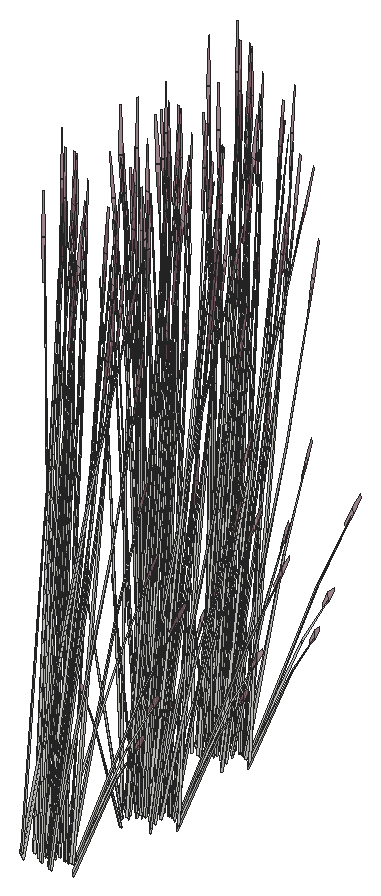
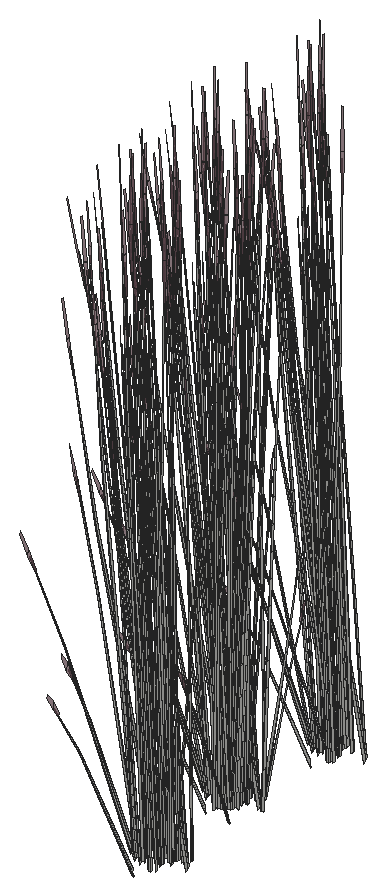
# SketchUp Ruby script. Lengths in inches.
U = 1.inch
M = Sketchup.active_model
def pt(a) = Geom::Point3d.new(a.map { |v| v * U })
def face(e, loops, mat)
  f = e.add_face(loops[0].map { |a| pt(a) })
  loops[1..].each { |l| e.add_face(l.map { |a| pt(a) }).erase! }
  f.material = f.back_material = mat if mat
  f
end
# faces: each face lists its corners as indices into pts; further lists are holes
def faces(e, pts, list, mat = nil) = list.each { |f| face(e, (f[0].is_a?(Array) ? f : [f]).map { |l| l.map { |i| pts[i] } }, mat) }
# xy, xz, yz: faces in a plane at the given z, y or x. An outline is a flat list of corners, or four numbers for a rectangle; further outlines are holes
def ring(l) = l.size == 4 ? [[l[0], l[1]], [l[2], l[1]], [l[2], l[3]], [l[0], l[3]]] : l.each_slice(2).to_a
def flat(e, list, mat, &to3) = list.each { |f| face(e, (f[0].is_a?(Array) ? f : [f]).map { |l| ring(l).map { |u, v| to3.(u, v) } }, mat) }
def xy(e, z, list, mat = nil) = flat(e, list, mat) { |x, y| [x, y, z] }
def xz(e, y, list, mat = nil) = flat(e, list, mat) { |x, z| [x, y, z] }
def yz(e, x, list, mat = nil) = flat(e, list, mat) { |y, z| [x, y, z] }
def lines(e, pts, list) = list.each { |a, b| e.add_line(pt(pts[a]), pt(pts[b])) }
# prism: a flat outline (further loops are holes) pulled along v
def prism(e, loops, v, mat = nil)
  f = face(e, loops, mat); d = Geom::Vector3d.new(v.map { |x| x * U })
  f.pushpull(f.normal.samedirection?(d) ? d.length : -d.length)
end
def box(e, o, s, mat = nil) = prism(e, [[o, [o[0] + s[0], o[1], o[2]], [o[0] + s[0], o[1] + s[1], o[2]], [o[0], o[1] + s[1], o[2]]]], [0, 0, s[2]], mat)
def at(x, y, z, deg = 0) = Geom::Transformation.translation(pt([x, y, z])) * Geom::Transformation.rotation(ORIGIN, Z_AXIS, deg.degrees)
def axes(o, x, y, z) = Geom::Transformation.new([*x, 0, *y, 0, *z, 0, *pt(o).to_a, 1])
def part(name) = M.definitions.add(name)
# library, detail: a bought-in or finely detailed component or shape, given as its bounding box
def library(name, o, s) = part(name).tap { |d| box(d.entities, o, s) }
def detail(e, o, s) = box(e.add_group.entities, o, s)
def put(e, d, t, mat = nil) = e.add_instance(d, t).tap { |i| i.material = mat if mat }
def group(e, t, mat = nil) = e.add_group.tap { |g| g.transformation = t; g.material = mat if mat }.entities
root = M.entities
M.materials.add("LightPink_Translucent").color = [144, 107, 117]
M.materials["LightPink_Translucent"].alpha = 0.75
c1 = part("blade")
p = [[2.15,0.21,22],[0,0.17,0],[0.09,0.45,0],[2.18,0.31,22],[2.29,0.31,22],[0.38,0.45,0],
  [2.48,0.24,33],[2.49,0.24,33],[2.48,0.22,33]]
faces(c1.entities,p,[[0,1,2,3],[4,5,2,3],[6,3,4,7],[8,0,3,6]])
c2 = part("seeds")
p = [[0.3,-0.1,1.38],[-0.01,-0.03,1.59],[-0.01,-0.03,0.03],[0.14,-0.07,-0.07],[0.29,-0.03,3],[0.15,0.01,3.11]]
faces(c2.entities,p,[[0,1,2,3],[1,0,4,5]],"LightPink_Translucent")
c3 = part("blade with seeds")
put(c3.entities,c1,at(0,0,0))
put(c3.entities,c2,axes([2.4,0.25,30.99],[1.5799,-0.05474,1.17369],[-0.12525,1.92788,0.29478],[-0.07173,-0.02425,1.56792]))
put(root,c3,axes([334.97,422.4,50.19],[-0.47255,-0.19538,0.43871],[0.28245,-0.35034,0],[0.10763,0.0445,1.3917]))
put(root,c3,axes([333.91,423.16,50.09],[-0.41865,0.35461,0.40429],[-0.49737,-0.31303,0.15865],[0.10093,-0.03539,1.40366]))
put(root,c3,axes([333.18,422.58,50.1875],[-0.14586,0.38834,0.15589],[-0.53375,-0.1099,0.31002],[0.0922,-0.00189,1.41735]))
put(root,c3,axes([332.96,422.89,49.41],[-0.49699,0.15644,1.13921],[-0.15819,-0.44887,0.44265],[0.30518,0.00747,1.29573]))
put(root,c3,axes([334.29,423.01,50.3125],[0.09741,-0.34873,0.12794],[0.4759,0.06053,-0.36534],[0.08661,0.03581,1.11991]))
put(root,c3,axes([336.84,423.5,49.32],[-0.02639,-0.05932,1.55816],[0.18302,-0.34702,-0.23804],[0.18462,-0.00499,0.26541]))
put(root,c3,axes([334.09,423.1,50.4],[-0.30332,-0.32798,0.39531],[0.45944,-0.23096,-0.19025],[0.09816,0.04058,1.26923]))
put(root,c3,axes([334.25,423.12,50.36],[0.50979,-0.25942,-0.25709],[0.339,0.36656,-0.44182],[0.12578,0.03723,1.41118]))
put(root,c3,axes([335.53,422.43,49.78],[0.47255,0.19538,-0.43871],[-0.28245,0.35034,0],[0.10763,0.0445,1.3917]))
put(root,c3,axes([334.63,423.55,49.95],[0.56491,0,0],[0,0.40454,0],[0,0,1.5764]))
put(root,c3,axes([334.79,422.6,50.1875],[-0.54257,0.10371,0.15589],[-0.13397,-0.38597,0.31002],[0.04839,0.05624,1.41735]))
put(root,c3,axes([335.4,422.58,49.79],[0.11861,0.34048,-0.27372],[-0.47106,0.09668,0.27372],[0.09497,0.03926,1.22797]))
put(root,c3,axes([334.45,423.34,50.1],[-0.63817,-0.08233,0.43472],[0.12987,-0.46497,0.17059],[0.09326,0.0449,1.50931]))
put(root,c3,axes([334.56,424.44,49.93],[0.53009,-0.13258,-0.16963],[0.18627,0.38191,0.00007],[0.05851,-0.01465,1.53656]))
put(root,c3,axes([334.62,423.72,49.96],[0.35245,0.2524,0],[-0.35245,0.2524,0],[0,0,1.49564]))
put(root,c3,axes([335.58,423.61,50.1875],[-0.39671,-0.28463,0.15589],[0.39978,-0.27607,0.31002],[-0.04381,0.05813,1.41735]))
put(root,c3,axes([334.84,423.18,49.82],[0.52523,0.06406,-0.55095],[-0.11084,0.39517,-0.1446],[0.15674,0.04788,1.21613]))
put(root,c3,axes([334.62,423.42,50.4],[0.24498,-0.3521,0.39531],[0.50902,0.16945,-0.19025],[0,0.08116,1.26923]))
put(root,c3,axes([334.52,423.625,50.03],[0,0.45191,-0.04981],[-0.63136,0,0],[0,0.0142,1.58489]))
put(root,c3,axes([334.57,423.31,49.95],[0.30332,0.32798,-0.39531],[-0.45944,0.23096,0.19025],[0.09816,0.04058,1.26923]))
put(root,c3,axes([335.9,423.62,50.19],[0,-0.39075,0.43871],[0.56491,0,0],[0,0.089,1.3917]))
put(root,c3,axes([334.83,423.5,50.3125],[0.47043,-0.11396,0.12794],[0.16474,0.32541,-0.36534],[0,0.07162,1.11991]))
put(root,c3,axes([336.58,424.3,50.29],[-0.1216,-0.0961,1.26356],[0.15822,-0.31792,-0.27174],[0.24603,0.04307,0.54024]))
put(root,c3,axes([334.4,424.65,49.95],[0.50902,0.17543,0],[-0.24498,0.36452,0],[0,0,1.54589]))
put(root,c3,axes([334.22,424.5,50.02],[0.21952,0.44891,-0.05313],[-0.62724,0.1573,0],[0.00767,0.01568,1.52132]))
put(root,c3,axes([336.29,423.6875,50.1],[0.63136,0,0],[0,0.43672,-0.456],[0,0.09947,1.44655]))
put(root,c3,axes([336.03,423.91,49.94],[-0.63105,-0.00312,-0.04397],[0,-0.43672,0.44129],[-0.01983,0.09942,1.3992]))
put(root,c3,axes([334.67,423.53,50.36],[0.56863,0.18645,-0.25709],[-0.2738,0.39352,-0.44182],[0.01787,0.09662,1.41118]))
put(root,c3,axes([335.9,423.97,49.79],[-0.35245,0.2438,-0.27372],[-0.35245,-0.2438,0.27372],[0,0.07853,1.22797]))
put(root,c3,axes([334.61,423.82,49.95],[-0.24498,0.3521,-0.39531],[-0.50902,-0.16945,0.19025],[0,0.08116,1.26923]))
put(root,c3,axes([336.15,423.98,49.78],[0,0.39075,-0.43871],[-0.56491,0,0],[0,0.089,1.3917]))
put(root,c3,axes([335.51,425.21,49.32],[0.03679,-0.05641,1.55816],[0.46313,-0.16615,-0.23804],[0.14041,0.08599,0.26541]))
put(root,c3,axes([334.9,423.93,49.85],[0.18514,0.35777,-0.61156],[-0.53331,0.12885,-0.16051],[0.02046,0.12115,1.3499]))
put(root,c3,axes([335.47,425.3,50.36],[-0.32378,-0.01225,0.92831],[0.21383,-0.26028,0.51254],[0.12791,0.09247,0.72818]))
put(root,c3,axes([334.42,424.67,50.29],[0.00891,-0.12953,1.26356],[0.4258,-0.14469,-0.27174],[0.13144,0.15503,0.54024]))
put(root,c3,axes([336.36,431.3,50.29],[-0.14352,0.07909,1.26356],[-0.42983,-0.13843,-0.27174],[0.07968,-0.17216,0.54024]))
put(root,c3,axes([335.29,430.87,49.32],[-0.08469,0.01408,1.55816],[-0.46834,-0.15847,-0.23804],[0.00786,-0.13218,0.26541]))
put(root,c3,axes([337.36,431.54,49.32],[-0.07557,-0.03078,1.55816],[-0.19412,-0.34391,-0.23804],[0.13095,-0.09333,0.26541]))
put(root,c3,axes([334.51,431.62,50.1],[-0.31568,-0.39156,0],[0.52815,-0.21836,-0.456],[0.12029,-0.04973,1.44655]))
put(root,c3,axes([335.2,431.14,49.88],[-0.34892,0.22417,-0.0344],[-0.3197,-0.24551,-0.15595],[-0.02251,-0.06957,0.51438]))
put(root,c3,axes([334.93,431.55,49.78],[0.47255,-0.19538,-0.43871],[0.28245,0.35034,0],[0.10763,-0.0445,1.3917]))
put(root,c3,axes([337.74,432.23,50.29],[-0.18038,-0.01157,1.26356],[-0.18479,-0.31048,-0.27174],[0.22159,-0.08783,0.54024]))
put(root,c3,axes([335.49,432.36,49.82],[0.34009,-0.2937,-0.55095],[0.42248,0.26632,-0.1446],[0.13628,-0.07327,1.21613]))
put(root,c3,axes([334.9,432.87,49.95],[0.24498,-0.3521,-0.39531],[0.50902,0.16945,0.19025],[0,-0.08116,1.26923]))
put(root,c3,axes([335.125,432.7,50.36],[-0.05884,-0.44587,-0.25709],[0.6128,-0.02696,-0.44182],[0.10791,-0.05939,1.41118]))
put(root,c3,axes([333.61,432.72,49.79],[0.35245,-0.2438,-0.27372],[0.35245,0.2438,0.27372],[0,-0.07853,1.22797]))
put(root,c3,axes([335.05,431.71,49.79],[0.47106,0.09668,-0.27372],[-0.11861,0.34048,0.27372],[0.09497,-0.03926,1.22797]))
put(root,c3,axes([335.21,433.05,50.15],[0.56891,0.18939,0.21263],[-0.2738,0.39352,0.44182],[0,-0.09071,1.41855]))
put(root,c3,axes([335.02,432.78,50.4],[-0.54829,0.02412,0.39531],[-0.04958,-0.40041,-0.19025],[0.09816,-0.04058,1.26923]))
put(root,c3,axes([336.83,431.71,50.1],[0.31568,-0.39156,0],[0.52815,0.21836,-0.456],[0.12029,0.04973,1.44655]))
put(root,c3,axes([335,432.93,50.09],[0.21952,0.43694,0.40429],[-0.62724,0.15194,0.15865],[0.00767,-0.08029,1.40366]))
put(root,c3,axes([338.07,433.26,49.75],[-0.3252,0.04689,1.25103],[-0.05176,-0.37326,0.07161],[0.22777,-0.0565,0.71188]))
put(root,c3,axes([338.67,432.93,50],[-0.31304,-0.24986,-0.05733],[0.34284,-0.22894,-0.25992],[0.09714,-0.01612,0.85731]))
put(root,c3,axes([334.89,433.27,50.4],[-0.24498,0.3521,0.39531],[-0.50902,-0.16945,-0.19025],[0,-0.08116,1.26923]))
put(root,c3,axes([335.79,432.96,49.95],[0,-0.45213,0],[0.63136,0,0],[0,0,1.58567]))
put(root,c3,axes([336.56,431.92,50.19],[-0.47255,-0.19538,0.43871],[0.28245,-0.35034,0],[0.10763,0.0445,1.3917]))
put(root,c3,axes([335.49,432.68,50.09],[-0.41865,0.35461,0.40429],[-0.49737,-0.31303,0.15865],[0.10093,-0.03539,1.40366]))
put(root,c3,axes([335.95,433.3125,50.03],[-0.46965,-0.33633,-0.05417],[0.46994,-0.33653,0],[-0.0164,-0.01174,1.55135]))
put(root,c3,axes([334.77,432.09,50.1875],[-0.14586,0.38834,0.15589],[-0.53375,-0.1099,0.31002],[0.0922,-0.00189,1.41735]))
put(root,c3,axes([334.55,432.41,49.41],[-0.49699,0.15644,1.13921],[-0.15819,-0.44887,0.44265],[0.30518,0.00747,1.29573]))
put(root,c3,axes([335.88,432.53,50.3125],[0.09741,-0.34873,0.12794],[0.4759,0.06053,-0.36534],[0.08661,0.03581,1.11991]))
put(root,c3,axes([335.06,433.35,50.09],[0.63817,0.08233,0.40429],[-0.12987,0.46497,0.15865],[-0.09326,-0.0449,1.40366]))
put(root,c3,axes([338.43,433.02,49.32],[-0.02639,-0.05932,1.55816],[0.18302,-0.34702,-0.23804],[0.18462,-0.00499,0.26541]))
put(root,c3,axes([335.68,432.62,50.4],[-0.30332,-0.32798,0.39531],[0.45944,-0.23096,-0.19025],[0.09816,0.04058,1.26923]))
put(root,c3,axes([334.72,434.1,50.1875],[0.54257,-0.10371,0.15589],[0.13397,0.38597,0.31002],[-0.04839,-0.05624,1.41735]))
put(root,c3,axes([335.83,432.64,50.36],[0.50979,-0.25942,-0.25709],[0.339,0.36656,-0.44182],[0.12578,0.03723,1.41118]))
put(root,c3,axes([337.12,431.95,49.78],[0.47255,0.19538,-0.43871],[-0.28245,0.35034,0],[0.10763,0.0445,1.3917]))
put(root,c3,axes([336.22,433.0625,49.95],[0.56491,0,0],[0,0.40454,0],[0,0,1.5764]))
put(root,c3,axes([336.38,432.12,50.1875],[-0.54257,0.10371,0.15589],[-0.13397,-0.38597,0.31002],[0.04839,0.05624,1.41735]))
put(root,c3,axes([336.99,432.1,49.79],[0.11861,0.34048,-0.27372],[-0.47106,0.09668,0.27372],[0.09497,0.03926,1.22797]))
put(root,c3,axes([336.04,432.86,50.1],[-0.63817,-0.08233,0.43472],[0.12987,-0.46497,0.17059],[0.09326,0.0449,1.50931]))
put(root,c3,axes([335.53,434.01,49.95],[-0.16474,-0.33688,0],[0.47043,-0.11798,0],[0,0,1.36402]))
put(root,c3,axes([336.15,433.96,49.93],[0.53009,-0.13258,-0.16963],[0.18627,0.38191,0.00007],[0.05851,-0.01465,1.53656]))
put(root,c3,axes([336.33,434.12,50.1875],[0.14586,-0.38834,0.15589],[0.53375,0.1099,0.31002],[-0.0922,0.00189,1.41735]))
put(root,c3,axes([336.21,433.24,49.96],[0.35245,0.2524,0],[-0.35245,0.2524,0],[0,0,1.49564]))
put(root,c3,axes([337.16,433.13,50.1875],[-0.39671,-0.28463,0.15589],[0.39978,-0.27607,0.31002],[-0.04381,0.05813,1.41735]))
put(root,c3,axes([336.43,432.7,49.82],[0.52523,0.06406,-0.55095],[-0.11084,0.39517,-0.1446],[0.15674,0.04788,1.21613]))
put(root,c3,axes([335.41,434.16,49.94],[-0.50902,-0.17543,0],[0.24498,-0.36452,0],[0,0,1.43768]))
put(root,c3,axes([336.2,432.94,50.4],[0.24498,-0.3521,0.39531],[0.50902,0.16945,-0.19025],[0,0.08116,1.26923]))
put(root,c3,axes([336.11,433.14,50.03],[0,0.45191,-0.04981],[-0.63136,0,0],[0,0.0142,1.58489]))
put(root,c3,axes([336.16,432.82,49.95],[0.30332,0.32798,-0.39531],[-0.45944,0.23096,0.19025],[0.09816,0.04058,1.26923]))
put(root,c3,axes([337.49,433.14,50.19],[0,-0.39075,0.43871],[0.56491,0,0],[0,0.089,1.3917]))
put(root,c3,axes([336.07,433.43,50.4],[0.54829,-0.02412,0.39531],[0.04958,0.40041,-0.19025],[-0.09816,0.04058,1.26923]))
put(root,c3,axes([336.42,433.02,50.3125],[0.47043,-0.11396,0.12794],[0.16474,0.32541,-0.36534],[0,0.07162,1.11991]))
put(root,c3,axes([338.16,433.82,50.29],[-0.1216,-0.0961,1.26356],[0.15822,-0.31792,-0.27174],[0.24603,0.04307,0.54024]))
put(root,c3,axes([335.99,434.17,49.95],[0.50902,0.17543,0],[-0.24498,0.36452,0],[0,0,1.54589]))
put(root,c3,axes([336.08,433.6,50.3125],[0.37303,0.23477,0.12794],[-0.31115,0.26487,-0.36534],[-0.08661,0.03581,1.11991]))
put(root,c3,axes([336.48,434.33,50.19],[0.47255,-0.19538,0.43871],[0.28245,0.35034,0],[-0.10763,0.0445,1.3917]))
put(root,c3,axes([335.81,434.02,50.02],[0.21952,0.44891,-0.05313],[-0.62724,0.1573,0],[0.00767,0.01568,1.52132]))
put(root,c3,axes([337.875,433.21,50.1],[0.63136,0,0],[0,0.43672,-0.456],[0,0.09947,1.44655]))
put(root,c3,axes([337.62,433.43,49.94],[-0.63105,-0.00312,-0.04397],[0,-0.43672,0.44129],[-0.01983,0.09942,1.3992]))
put(root,c3,axes([336.26,433.05,50.36],[0.56863,0.18645,-0.25709],[-0.2738,0.39352,-0.44182],[0.01787,0.09662,1.41118]))
put(root,c3,axes([337.49,433.49,49.79],[-0.35245,0.2438,-0.27372],[-0.35245,-0.2438,0.27372],[0,0.07853,1.22797]))
put(root,c3,axes([336.19,433.34,49.95],[-0.24498,0.3521,-0.39531],[-0.50902,-0.16945,0.19025],[0,0.08116,1.26923]))
put(root,c3,axes([336.21,434.35,50.06],[0.63212,0.12701,0.27176],[-0.15814,0.45398,-0.32244],[-0.10462,0.05682,1.45692]))
put(root,c3,axes([337.73,433.5,49.78],[0,0.39075,-0.43871],[-0.56491,0,0],[0,0.089,1.3917]))
put(root,c3,axes([336.59,434.6,50.1],[0.31568,0.39156,0],[-0.52815,0.21836,-0.456],[-0.12029,0.04973,1.44655]))
put(root,c3,axes([337.09,434.73,49.32],[0.03679,-0.05641,1.55816],[0.46313,-0.16615,-0.23804],[0.14041,0.08599,0.26541]))
put(root,c3,axes([336.48,433.45,49.85],[0.18514,0.35777,-0.61156],[-0.53331,0.12885,-0.16051],[0.02046,0.12115,1.3499]))
put(root,c3,axes([337.06,434.82,50.36],[-0.32378,-0.01225,0.92831],[0.21383,-0.26028,0.51254],[0.12791,0.09247,0.72818]))
put(root,c3,axes([336,434.19,50.29],[0.00891,-0.12953,1.26356],[0.4258,-0.14469,-0.27174],[0.13144,0.15503,0.54024]))
put(root,c3,axes([334.93,434.72,49.32],[0.08172,-0.02126,1.55816],[0.49154,0.11703,-0.23804],[0.01437,0.1319,0.26541]))
put(root,c3,axes([334.77,441.17,50.29],[-0.14352,0.07909,1.26356],[-0.42983,-0.13843,-0.27174],[0.07968,-0.17216,0.54024]))
put(root,c3,axes([335.77,441.41,49.32],[-0.07557,-0.03078,1.55816],[-0.19412,-0.34391,-0.23804],[0.13095,-0.09333,0.26541]))
put(root,c3,axes([332.92,441.48,50.1],[-0.31568,-0.39156,0],[0.52815,-0.21836,-0.456],[0.12029,-0.04973,1.44655]))
put(root,c3,axes([333.35,441.42,49.78],[0.47255,-0.19538,-0.43871],[0.28245,0.35034,0],[0.10763,-0.0445,1.3917]))
put(root,c3,axes([336.15,442.1,50.29],[-0.18038,-0.01157,1.26356],[-0.18479,-0.31048,-0.27174],[0.22159,-0.08783,0.54024]))
put(root,c3,axes([333.91,442.22,49.82],[0.34009,-0.2937,-0.55095],[0.42248,0.26632,-0.1446],[0.13628,-0.07327,1.21613]))
put(root,c3,axes([333.54,442.5625,50.36],[-0.05884,-0.44587,-0.25709],[0.6128,-0.02696,-0.44182],[0.10791,-0.05939,1.41118]))
put(root,c3,axes([333.46,441.58,49.79],[0.47106,0.09668,-0.27372],[-0.11861,0.34048,0.27372],[0.09497,-0.03926,1.22797]))
put(root,c3,axes([333.62,442.91,50.15],[0.56891,0.18939,0.21263],[-0.2738,0.39352,0.44182],[0,-0.09071,1.41855]))
put(root,c3,axes([333.44,442.65,50.4],[-0.54829,0.02412,0.39531],[-0.04958,-0.40041,-0.19025],[0.09816,-0.04058,1.26923]))
put(root,c3,axes([335.24,441.58,50.1],[0.31568,-0.39156,0],[0.52815,0.21836,-0.456],[0.12029,0.04973,1.44655]))
put(root,c3,axes([336.49,443.13,49.75],[-0.3252,0.04689,1.25103],[-0.05176,-0.37326,0.07161],[0.22777,-0.0565,0.71188]))
put(root,c3,axes([337.08,442.8,50],[-0.31304,-0.24986,-0.05733],[0.34284,-0.22894,-0.25992],[0.09714,-0.01612,0.85731]))
put(root,c3,axes([334.21,442.83,49.95],[0,-0.45213,0],[0.63136,0,0],[0,0,1.58567]))
put(root,c3,axes([334.97,441.79,50.19],[-0.47255,-0.19538,0.43871],[0.28245,-0.35034,0],[0.10763,0.0445,1.3917]))
put(root,c3,axes([333.91,442.55,50.09],[-0.41865,0.35461,0.40429],[-0.49737,-0.31303,0.15865],[0.10093,-0.03539,1.40366]))
put(root,c3,axes([333.18,441.96,50.1875],[-0.14586,0.38834,0.15589],[-0.53375,-0.1099,0.31002],[0.0922,-0.00189,1.41735]))
put(root,c3,axes([332.96,442.28,49.41],[-0.49699,0.15644,1.13921],[-0.15819,-0.44887,0.44265],[0.30518,0.00747,1.29573]))
put(root,c3,axes([334.29,442.39,50.3125],[0.09741,-0.34873,0.12794],[0.4759,0.06053,-0.36534],[0.08661,0.03581,1.11991]))
put(root,c3,axes([336.84,442.88,49.32],[-0.02639,-0.05932,1.55816],[0.18302,-0.34702,-0.23804],[0.18462,-0.00499,0.26541]))
put(root,c3,axes([334.09,442.48,50.4],[-0.30332,-0.32798,0.39531],[0.45944,-0.23096,-0.19025],[0.09816,0.04058,1.26923]))
put(root,c3,axes([334.25,442.51,50.36],[0.50979,-0.25942,-0.25709],[0.339,0.36656,-0.44182],[0.12578,0.03723,1.41118]))
put(root,c3,axes([335.53,441.82,49.78],[0.47255,0.19538,-0.43871],[-0.28245,0.35034,0],[0.10763,0.0445,1.3917]))
put(root,c3,axes([334.63,442.93,49.95],[0.56491,0,0],[0,0.40454,0],[0,0,1.5764]))
put(root,c3,axes([334.79,441.98,50.1875],[-0.54257,0.10371,0.15589],[-0.13397,-0.38597,0.31002],[0.04839,0.05624,1.41735]))
put(root,c3,axes([335.4,441.96,49.79],[0.11861,0.34048,-0.27372],[-0.47106,0.09668,0.27372],[0.09497,0.03926,1.22797]))
put(root,c3,axes([334.45,442.73,50.1],[-0.63817,-0.08233,0.43472],[0.12987,-0.46497,0.17059],[0.09326,0.0449,1.50931]))
put(root,c3,axes([334.56,443.83,49.93],[0.53009,-0.13258,-0.16963],[0.18627,0.38191,0.00007],[0.05851,-0.01465,1.53656]))
put(root,c3,axes([334.62,443.1,49.96],[0.35245,0.2524,0],[-0.35245,0.2524,0],[0,0,1.49564]))
put(root,c3,axes([335.58,442.99,50.1875],[-0.39671,-0.28463,0.15589],[0.39978,-0.27607,0.31002],[-0.04381,0.05813,1.41735]))
put(root,c3,axes([334.84,442.56,49.82],[0.52523,0.06406,-0.55095],[-0.11084,0.39517,-0.1446],[0.15674,0.04788,1.21613]))
put(root,c3,axes([334.62,442.81,50.4],[0.24498,-0.3521,0.39531],[0.50902,0.16945,-0.19025],[0,0.08116,1.26923]))
put(root,c3,axes([334.52,443.01,50.03],[0,0.45191,-0.04981],[-0.63136,0,0],[0,0.0142,1.58489]))
put(root,c3,axes([334.57,442.69,49.95],[0.30332,0.32798,-0.39531],[-0.45944,0.23096,0.19025],[0.09816,0.04058,1.26923]))
put(root,c3,axes([335.9,443.01,50.19],[0,-0.39075,0.43871],[0.56491,0,0],[0,0.089,1.3917]))
put(root,c3,axes([334.83,442.89,50.3125],[0.47043,-0.11396,0.12794],[0.16474,0.32541,-0.36534],[0,0.07162,1.11991]))
put(root,c3,axes([336.58,443.68,50.29],[-0.1216,-0.0961,1.26356],[0.15822,-0.31792,-0.27174],[0.24603,0.04307,0.54024]))
put(root,c3,axes([334.4,444.03,49.95],[0.50902,0.17543,0],[-0.24498,0.36452,0],[0,0,1.54589]))
put(root,c3,axes([334.22,443.89,50.02],[0.21952,0.44891,-0.05313],[-0.62724,0.1573,0],[0.00767,0.01568,1.52132]))
put(root,c3,axes([336.29,443.07,50.1],[0.63136,0,0],[0,0.43672,-0.456],[0,0.09947,1.44655]))
put(root,c3,axes([336.03,443.3,49.94],[-0.63105,-0.00312,-0.04397],[0,-0.43672,0.44129],[-0.01983,0.09942,1.3992]))
put(root,c3,axes([334.67,442.92,50.36],[0.56863,0.18645,-0.25709],[-0.2738,0.39352,-0.44182],[0.01787,0.09662,1.41118]))
put(root,c3,axes([335.9,443.36,49.79],[-0.35245,0.2438,-0.27372],[-0.35245,-0.2438,0.27372],[0,0.07853,1.22797]))
put(root,c3,axes([334.61,443.21,49.95],[-0.24498,0.3521,-0.39531],[-0.50902,-0.16945,0.19025],[0,0.08116,1.26923]))
put(root,c3,axes([336.15,443.37,49.78],[0,0.39075,-0.43871],[-0.56491,0,0],[0,0.089,1.3917]))
put(root,c3,axes([335.51,444.6,49.32],[0.03679,-0.05641,1.55816],[0.46313,-0.16615,-0.23804],[0.14041,0.08599,0.26541]))
